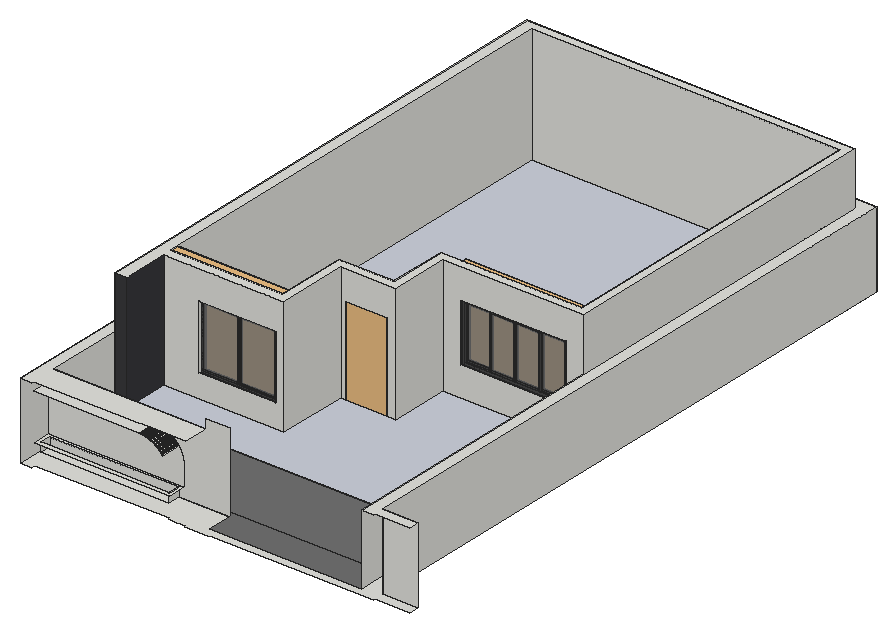
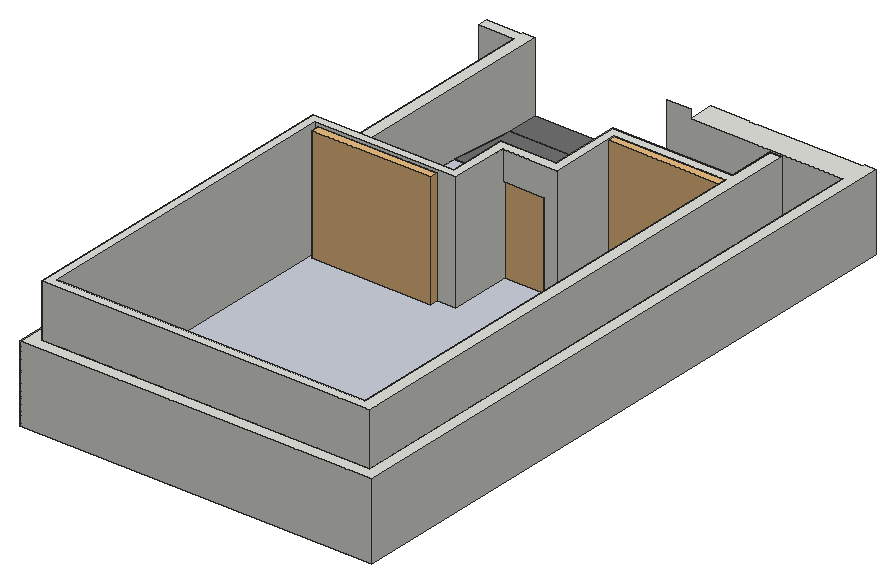
# SketchUp Ruby script. Lengths in inches.
U = 1.inch
M = Sketchup.active_model
def pt(a) = Geom::Point3d.new(a.map { |v| v * U })
def face(e, loops, mat)
  f = e.add_face(loops[0].map { |a| pt(a) })
  loops[1..].each { |l| e.add_face(l.map { |a| pt(a) }).erase! }
  f.material = f.back_material = mat if mat
  f
end
# faces: each face lists its corners as indices into pts; further lists are holes
def faces(e, pts, list, mat = nil) = list.each { |f| face(e, (f[0].is_a?(Array) ? f : [f]).map { |l| l.map { |i| pts[i] } }, mat) }
# xy, xz, yz: faces in a plane at the given z, y or x. An outline is a flat list of corners, or four numbers for a rectangle; further outlines are holes
def ring(l) = l.size == 4 ? [[l[0], l[1]], [l[2], l[1]], [l[2], l[3]], [l[0], l[3]]] : l.each_slice(2).to_a
def flat(e, list, mat, &to3) = list.each { |f| face(e, (f[0].is_a?(Array) ? f : [f]).map { |l| ring(l).map { |u, v| to3.(u, v) } }, mat) }
def xy(e, z, list, mat = nil) = flat(e, list, mat) { |x, y| [x, y, z] }
def xz(e, y, list, mat = nil) = flat(e, list, mat) { |x, z| [x, y, z] }
def yz(e, x, list, mat = nil) = flat(e, list, mat) { |y, z| [x, y, z] }
def lines(e, pts, list) = list.each { |a, b| e.add_line(pt(pts[a]), pt(pts[b])) }
# prism: a flat outline (further loops are holes) pulled along v
def prism(e, loops, v, mat = nil)
  f = face(e, loops, mat); d = Geom::Vector3d.new(v.map { |x| x * U })
  f.pushpull(f.normal.samedirection?(d) ? d.length : -d.length)
end
def box(e, o, s, mat = nil) = prism(e, [[o, [o[0] + s[0], o[1], o[2]], [o[0] + s[0], o[1] + s[1], o[2]], [o[0], o[1] + s[1], o[2]]]], [0, 0, s[2]], mat)
def at(x, y, z, deg = 0) = Geom::Transformation.translation(pt([x, y, z])) * Geom::Transformation.rotation(ORIGIN, Z_AXIS, deg.degrees)
def axes(o, x, y, z) = Geom::Transformation.new([*x, 0, *y, 0, *z, 0, *pt(o).to_a, 1])
def part(name) = M.definitions.add(name)
# library, detail: a bought-in or finely detailed component or shape, given as its bounding box
def library(name, o, s) = part(name).tap { |d| box(d.entities, o, s) }
def detail(e, o, s) = box(e.add_group.entities, o, s)
def put(e, d, t, mat = nil) = e.add_instance(d, t).tap { |i| i.material = mat if mat }
def group(e, t, mat = nil) = e.add_group.tap { |g| g.transformation = t; g.material = mat if mat }.entities
root = M.entities
M.materials.add("1432 AP 8245 TAR ROAD").color = [57, 57, 60]
M.materials.add("[Granite Tile]").color = [112, 112, 112]
M.materials.add("[Marble Carrara Floor Tile]").color = [204, 208, 219]
M.materials.add("[Steel Brushed Stainless]").color = [71, 71, 71]
M.materials.add("[Translucent Glass Gray]").color = [128, 128, 128]
M.materials["[Translucent Glass Gray]"].alpha = 0.5
M.materials.add("[Translucent_Glass_Gray]").color = [128, 128, 128]
M.materials["[Translucent_Glass_Gray]"].alpha = 0.5
c1 = library("Component",[0,-3.14,-0.03],[53.55,5.67,83.24])
c2 = part("Window frame")
prism(c2.entities,[[[0,70.87,0],[0,0,0],[0,0,47.24],[0,70.87,47.24]],[[0,1.97,1.97],[0,68.9,1.97],[0,68.9,45.28],[0,1.97,45.28]]],[7.875,0,0])
c3 = part("Window sash")
xy(c3.entities,0,[[0,0,3.9375,16.73]])
xy(c3.entities,0.98,[[0,0.98,1.77,15.75],[1.77,0.98,2.85,15.75],[2.85,0.98,3.9375,15.75]])
xy(c3.entities,42.32,[[0,0.98,1.77,15.75],[1.77,0.98,2.85,15.75],[2.85,0.98,3.9375,15.75]])
xy(c3.entities,43.31,[[0,0,3.9375,16.73]])
xz(c3.entities,0,[[0,0,3.9375,43.31]])
xz(c3.entities,0.98,[[0,0.98,1.77,42.32],[1.77,0.98,2.85,42.32],[2.85,0.98,3.9375,42.32]])
xz(c3.entities,15.75,[[0,0.98,1.77,42.32],[1.77,0.98,2.85,42.32],[2.85,0.98,3.9375,42.32]])
xz(c3.entities,16.73,[[0,0,3.9375,43.31]])
yz(c3.entities,0,[[[0,0,16.73,43.31],[0.98,0.98,15.75,42.32]]])
yz(c3.entities,1.77,[[0.98,0.98,15.75,42.32]],"[Translucent_Glass_Gray]")
yz(c3.entities,2.85,[[0.98,0.98,15.75,42.32]],"[Translucent_Glass_Gray]")
yz(c3.entities,3.9375,[[[0,0,16.73,43.31],[0.98,0.98,15.75,42.32]]])
c4 = part("simple window")
p = [[0,68.9,1.97],[0,35.43,1.97]]
lines(c4.entities,p,[[0,1]])
put(c4.entities,c2,at(0,0,0),"[Steel Brushed Stainless]")
put(c4.entities,c3,axes([1.14,52.17,1.97],[0.71,0,0],[0,1,0],[0,0,1]),"[Steel Brushed Stainless]")
put(c4.entities,c3,axes([1.14,1.97,1.97],[0.71,0,0],[0,1,0],[0,0,1]),"[Steel Brushed Stainless]")
put(c4.entities,c3,axes([3.9375,18.7,1.97],[0.71,0,0],[0,1,0],[0,0,1]),"[Steel Brushed Stainless]")
put(c4.entities,c3,axes([3.9375,35.43,1.97],[0.71,0,0],[0,1,0],[0,0,1]),"[Steel Brushed Stainless]")
c5 = library("Curtains",[0,0,0],[121.73,8.19,117.22])
c6 = part("1")
prism(c6.entities,[[[36.75,0,63],[36.75,0,0],[0,0,0],[0,0,63]],[[1,0,1],[35.75,0,1],[35.75,0,62],[1,0,62]]],[0,-1.25,0])
g1 = group(c6.entities,at(1,-0.4375,1),"[Translucent Glass Gray]")
box(g1,[0,-0.47,0],[34.75,0.47,61])
xy(root,-12,[[0,58,0,704,360,704,360,72,396,72,396,62,360,62,360,60,192,60,192,58,168,58,168,60,160,60,160,60.5,159,60.5,159,60,150,60,150,62,12,62,12,58]])
xy(root,-6,[[12,92,348,164],[12,164,348,692]])
xy(root,-6,[[192,60,348,60,348,92,12,92,12,86,192,86]],"[Granite Tile]")
xy(root,0,[[15,65,147,77]])
xy(root,9,[[[12,62,150,80],[15,65,147,77]]])
xy(root,57,[[12,60,120,80],[120,60,120.39,80]])
xy(root,66,[[0,58,12,58,12,60,120,60,120,60.5,128.89,60.5,128.89,60,168,60,168,86,12,86,12,692,348,692,348,60,360,60,360,62,396,62,396,72,360,72,360,704,0,704]])
xz(root,72,[[360,-12,396,66]])
xz(root,77,[[15,0,147,9]])
xz(root,80,[[12,9,150,9,150,27.39,149.99,27.79,149.98,28.18,149.96,28.57,149.9375,28.96,149.91,29.35,149.875,29.75,149.84,30.14,149.74,30.92,149.69,31.3,149.57,32.08,149.5,32.47,149.42,32.85,149.34,33.24,149.26,33.62,149.08,34.38,148.98,34.76,148.875,35.14,148.76,35.52,148.65,35.9,148.41,36.64,148.15,37.38,148.01,37.75,147.86,38.12,147.72,38.48,147.5625,38.84,147.41,39.2,147.24,39.56,147.08,39.92,146.91,40.27,146.55,40.97,146.36,41.31,146.17,41.66,145.98,42,145.78,42.34,145.58,42.67,145.37,43.01,145.16,43.34,144.94,43.67,144.72,43.99,144.5,44.3125,144.27,44.63,144.04,44.95,143.56,45.57,143.3125,45.88,143.07,46.18,142.8125,46.48,142.56,46.78,142.29,47.07,142.03,47.36,141.76,47.65,141.49,47.93,140.93,48.49,140.65,48.76,140.36,49.03,140.07,49.29,139.78,49.56,139.48,49.8125,139.18,50.07,138.88,50.3125,138.57,50.56,137.95,51.04,137.63,51.27,137.3125,51.5,136.99,51.72,136.67,51.94,136.34,52.16,136.01,52.37,135.67,52.58,135.34,52.78,135,52.98,134.66,53.17,134.31,53.36,133.97,53.55,133.27,53.91,132.92,54.08,132.56,54.24,132.2,54.41,131.84,54.5625,131.48,54.72,131.12,54.86,130.75,55.01,130.38,55.15,129.64,55.41,128.9,55.65,128.52,55.76,128.14,55.875,127.76,55.98,127.38,56.08,126.62,56.26,126.24,56.34,125.85,56.42,125.47,56.5,125.08,56.57,124.3,56.69,123.92,56.74,123.14,56.84,122.75,56.875,122.35,56.91,121.96,56.9375,121.57,56.96,121.18,56.98,120.79,56.99,120.39,57,12,57]])
xz(root,86,[[12,-6,12,66,168,66,168,75,192,75,192,-6]])
xz(root,164,[[12,-6,348,0]])
xz(root,692,[[12,-6,348,66]])
xz(root,704,[[0,-12,360,66]])
yz(root,0,[[58,-12,704,66]])
yz(root,12,[[86,-6,92,-6,164,0,164,66,86,66],[92,-6,164,-6,164,0],[164,-6,692,66]])
yz(root,15,[[65,0,77,9]])
yz(root,147,[[65,0,77,9]])
yz(root,348,[[60,-6,60,66,692,66,692,-6,164,-6,164,0,92,-6],[92,-6,164,0,164,-6]])
yz(root,360,[[72,-12,704,66]])
p = [[348,92,-6],[348,164,0],[12,164,0],[12,92,-6],[144.27,80,44.63],[144.27,60,44.63],
  [144.04,60,44.95],[144.04,80,44.95],[143.8,60,45.26],[143.8,80,45.26],[143.56,60,45.57],[143.56,80,45.57],
  [143.3125,60,45.88],[143.3125,80,45.88],[143.07,60,46.18],[143.07,80,46.18],[142.8125,60,46.48],[142.8125,80,46.48],
  [142.56,60,46.78],[142.56,80,46.78],[142.29,60,47.07],[142.29,80,47.07],[142.03,60,47.36],[142.03,80,47.36],
  [141.76,60,47.65],[141.76,80,47.65],[141.49,60,47.93],[141.49,80,47.93],[141.21,60,48.21],[141.21,80,48.21],
  [140.93,60,48.49],[140.93,80,48.49],[140.65,60,48.76],[140.65,80,48.76],[140.36,60,49.03],[140.36,80,49.03],
  [140.07,60,49.29],[140.07,80,49.29],[139.78,60,49.56],[139.78,80,49.56],[139.48,60,49.8125],[139.48,80,49.8125],
  [139.18,60,50.07],[139.18,80,50.07],[138.88,60,50.3125],[138.88,80,50.3125],[138.57,60,50.56],[138.57,80,50.56],
  [138.26,60,50.8],[138.26,80,50.8],[137.95,60,51.04],[137.95,80,51.04],[137.63,60,51.27],[137.63,80,51.27],
  [137.3125,60,51.5],[137.3125,80,51.5],[136.99,60,51.72],[136.99,80,51.72],[136.67,60,51.94],[136.67,80,51.94],
  [136.34,60,52.16],[136.34,80,52.16],[136.01,60,52.37],[136.01,80,52.37],[135.67,60,52.58],[135.67,80,52.58],
  [135.34,60,52.78],[135.34,80,52.78],[135,60,52.98],[135,80,52.98],[134.66,60,53.17],[134.66,80,53.17],
  [134.31,60,53.36],[134.31,80,53.36],[133.97,60,53.55],[133.97,80,53.55],[133.62,60,53.73],[133.62,80,53.73],
  [133.27,60,53.91],[133.27,80,53.91],[132.92,60,54.08],[132.92,80,54.08],[132.56,60,54.24],[132.56,80,54.24],
  [132.2,60,54.41],[132.2,80,54.41],[131.84,60,54.5625],[131.84,80,54.5625],[131.48,60,54.72],[131.48,80,54.72],
  [131.12,60,54.86],[131.12,80,54.86],[130.75,60,55.01],[130.75,80,55.01],[130.38,60,55.15],[130.38,80,55.15],
  [130.01,60,55.28],[130.01,80,55.28],[129.64,60,55.41],[129.64,80,55.41],[129.27,60,55.53],[129.27,80,55.53],
  [128.9,60,55.65],[128.9,80,55.65],[128.52,60,55.76],[128.52,80,55.76],[128.14,60,55.875],[128.14,80,55.875],
  [127.76,60,55.98],[127.76,80,55.98],[127.38,60,56.08],[127.38,80,56.08],[127,60,56.17],[127,80,56.17],
  [126.62,60,56.26],[126.62,80,56.26],[126.24,80,56.34],[126.24,60,56.34],[125.85,60,56.42],[125.85,80,56.42],
  [125.47,60,56.5],[125.47,80,56.5],[125.08,60,56.57],[125.08,80,56.57],[124.69,80,56.63],[124.69,60,56.63],
  [124.3,60,56.69],[124.3,80,56.69],[123.92,80,56.74],[123.92,60,56.74],[123.53,60,56.79],[123.53,80,56.79],
  [123.14,80,56.84],[123.14,60,56.84],[122.75,60,56.875],[122.75,80,56.875],[121.96,80,56.9375],[121.96,60,56.9375],
  [121.57,60,56.96],[121.57,80,56.96],[122.35,80,56.91],[122.35,60,56.91],[120.79,80,56.99],[120.79,60,56.99],
  [120.39,60,57],[120.39,80,57],[121.18,80,56.98],[121.18,60,56.98]]
faces(root,p,[[0,1,2,3]],"[Granite Tile]")
faces(root,p,[[4,5,6,7],[7,6,8,9],[9,8,10,11],[11,10,12,13],[13,12,14,15],[15,14,16,17],[17,16,18,19],[19,18,20,21],
  [21,20,22,23],[23,22,24,25],[25,24,26,27],[27,26,28,29],[29,28,30,31],[31,30,32,33],[33,32,34,35],[35,34,36,37],
  [37,36,38,39],[39,38,40,41],[41,40,42,43],[43,42,44,45],[45,44,46,47],[47,46,48,49],[49,48,50,51],[51,50,52,53],
  [53,52,54,55],[55,54,56,57],[57,56,58,59],[59,58,60,61],[61,60,62,63],[63,62,64,65],[65,64,66,67],[67,66,68,69],
  [69,68,70,71],[71,70,72,73],[73,72,74,75],[75,74,76,77],[77,76,78,79],[79,78,80,81],[81,80,82,83],[83,82,84,85],
  [85,84,86,87],[87,86,88,89],[89,88,90,91],[91,90,92,93],[93,92,94,95],[95,94,96,97],[97,96,98,99],[99,98,100,101],
  [101,100,102,103],[103,102,104,105],[105,104,106,107],[107,106,108,109],[109,108,110,111],[111,110,112,113],[113,112,114,115],[116,117,118,119],
  [115,114,117,116],[119,118,120,121],[121,120,122,123],[124,125,126,127],[123,122,125,124],[128,129,130,131],[127,126,129,128],[132,133,134,135],
  [131,130,133,132],[136,137,138,139],[140,141,137,136],[135,134,141,140],[142,143,144,145],[146,147,143,142],[139,138,147,146]])
g2 = group(root,at(12,164,0))
xy(g2,-6,[[0,0,336,528]])
xy(g2,0,[[0,0,336,528]],"[Marble Carrara Floor Tile]")
xz(g2,0,[[0,-6,336,0]])
xz(g2,528,[[0,-6,336,0]])
yz(g2,0,[[0,-6,528,0]])
yz(g2,336,[[0,-6,528,0]])
g3 = group(root,at(12,212,0))
xy(g3,0,[[0,-48,0,480,336,480,336,132,192,132,192,72,183,72,183,141,327,141,327,471,12,471,12,9,126,9,126,81,141,81,141,72,135,72,135,0,12,0,12,-48]])
xy(g3,24,[[48,0,126,9]])
xy(g3,30,[[210,132,318,141]])
xy(g3,90,[[48,0,126,9],[141,72,183,81],[210,132,318,141]])
xy(g3,120,[[[0,-48,12,-48,12,0,135,0,135,72,192,72,192,132,336,132,336,480,0,480],[12,9,12,471,327,471,327,141,183,141,183,81,126,81,126,9]]])
xz(g3,-48,[[0,0,12,120]],"1432 AP 8245 TAR ROAD")
xz(g3,0,[[[12,0,135,120],[48,24,126,90]]])
xz(g3,9,[[12,0,12,120,126,120,126,90,48,90,48,24,126,24,126,0]])
xz(g3,72,[[135,0,141,0,141,90,183,90,183,0,192,0,192,120,135,120]])
xz(g3,81,[[126,0,126,120,183,120,183,90,141,90,141,0]])
xz(g3,132,[[[192,0,336,120],[210,30,318,90]]])
xz(g3,141,[[[183,0,327,120],[210,30,318,90]]])
xz(g3,471,[[12,0,327,120]])
xz(g3,480,[[0,0,336,120]])
yz(g3,0,[[-48,0,480,120]])
yz(g3,12,[[9,0,471,120]])
yz(g3,12,[[-48,0,0,120]],"1432 AP 8245 TAR ROAD")
yz(g3,48,[[0,24,9,90]])
yz(g3,126,[[9,0,81,120],[0,24,9,90]])
yz(g3,135,[[0,0,72,120]])
yz(g3,141,[[72,0,81,90]])
yz(g3,183,[[72,0,72,90,81,90,81,120,141,120,141,0]])
yz(g3,192,[[72,0,132,120]])
yz(g3,210,[[132,30,141,90]])
yz(g3,318,[[132,30,141,90]])
yz(g3,327,[[141,0,471,120]])
yz(g3,336,[[132,0,480,120]])
put(g3,c1,axes([141,75.14,0],[0.78433,0,0],[0,1,0],[0,0,1.0816]))
put(g3,c4,axes([210,138.8,30],[0,-0.61,0],[1.524,0,0],[0,0,1.27]))
put(g3,c5,at(201.92,141,0))
put(g3,c5,axes([12,9,2.78],[0.93652,0,0],[0,1,0],[0,0,1]))
g4 = group(g3,at(48,4,24),"[Steel Brushed Stainless]")
prism(g4,[[[0,0,66],[78,0,66],[78,0,0],[0,0,0]],[[38.25,0,64.5],[1.5,0,64.5],[1.5,0,1.5],[38.25,0,1.5]],[[39.75,0,64.5],[39.75,0,1.5],[76.5,0,1.5],[76.5,0,64.5]]],[0,-2,0])
put(g4,c6,at(1.5,0,1.5))
put(g4,c6,at(39.75,0,1.5))
